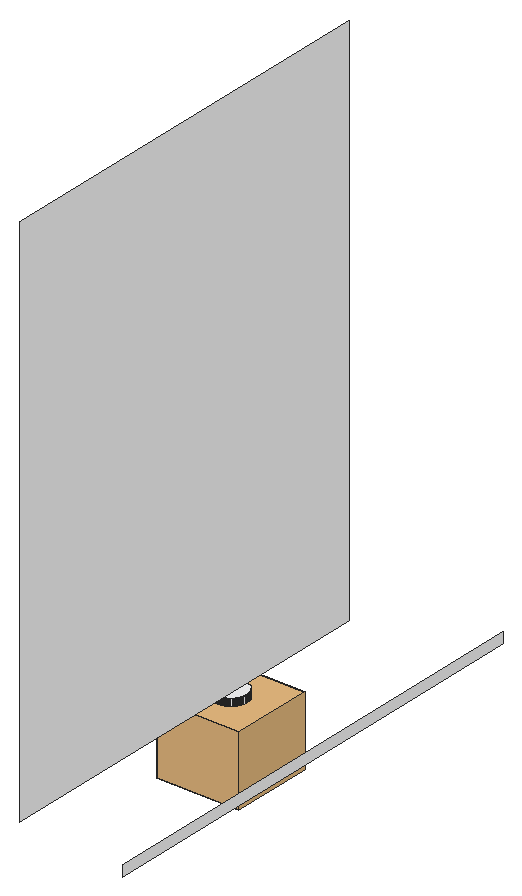
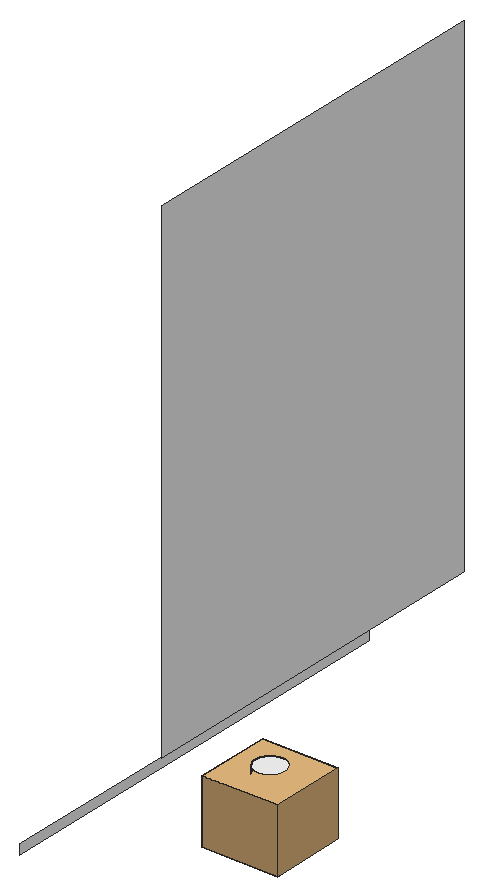
# SketchUp Ruby script. Lengths in inches.
U = 1.inch
M = Sketchup.active_model
def pt(a) = Geom::Point3d.new(a.map { |v| v * U })
def face(e, loops, mat)
  f = e.add_face(loops[0].map { |a| pt(a) })
  loops[1..].each { |l| e.add_face(l.map { |a| pt(a) }).erase! }
  f.material = f.back_material = mat if mat
  f
end
# faces: each face lists its corners as indices into pts; further lists are holes
def faces(e, pts, list, mat = nil) = list.each { |f| face(e, (f[0].is_a?(Array) ? f : [f]).map { |l| l.map { |i| pts[i] } }, mat) }
# xy, xz, yz: faces in a plane at the given z, y or x. An outline is a flat list of corners, or four numbers for a rectangle; further outlines are holes
def ring(l) = l.size == 4 ? [[l[0], l[1]], [l[2], l[1]], [l[2], l[3]], [l[0], l[3]]] : l.each_slice(2).to_a
def flat(e, list, mat, &to3) = list.each { |f| face(e, (f[0].is_a?(Array) ? f : [f]).map { |l| ring(l).map { |u, v| to3.(u, v) } }, mat) }
def xy(e, z, list, mat = nil) = flat(e, list, mat) { |x, y| [x, y, z] }
def xz(e, y, list, mat = nil) = flat(e, list, mat) { |x, z| [x, y, z] }
def yz(e, x, list, mat = nil) = flat(e, list, mat) { |y, z| [x, y, z] }
def lines(e, pts, list) = list.each { |a, b| e.add_line(pt(pts[a]), pt(pts[b])) }
# prism: a flat outline (further loops are holes) pulled along v
def prism(e, loops, v, mat = nil)
  f = face(e, loops, mat); d = Geom::Vector3d.new(v.map { |x| x * U })
  f.pushpull(f.normal.samedirection?(d) ? d.length : -d.length)
end
def box(e, o, s, mat = nil) = prism(e, [[o, [o[0] + s[0], o[1], o[2]], [o[0] + s[0], o[1] + s[1], o[2]], [o[0], o[1] + s[1], o[2]]]], [0, 0, s[2]], mat)
def at(x, y, z, deg = 0) = Geom::Transformation.translation(pt([x, y, z])) * Geom::Transformation.rotation(ORIGIN, Z_AXIS, deg.degrees)
def axes(o, x, y, z) = Geom::Transformation.new([*x, 0, *y, 0, *z, 0, *pt(o).to_a, 1])
def part(name) = M.definitions.add(name)
# library, detail: a bought-in or finely detailed component or shape, given as its bounding box
def library(name, o, s) = part(name).tap { |d| box(d.entities, o, s) }
def detail(e, o, s) = box(e.add_group.entities, o, s)
def put(e, d, t, mat = nil) = e.add_instance(d, t).tap { |i| i.material = mat if mat }
def group(e, t, mat = nil) = e.add_group.tap { |g| g.transformation = t; g.material = mat if mat }.entities
root = M.entities
M.materials.add("[Quartz Light Grey]").color = [251, 251, 252]
c1 = library("5",[-6.25,-6.25,-13.16],[15.58,15.58,13.16])
xy(root,119.5,[[207.84,250,207.76,250.01,207.6875,250.02,207.61,250.03,207.45,250.05,207.375,250.07,207.3,250.08,207.22,250.1,207.15,250.125,207.07,250.15,207,250.17,206.92,250.2,206.71,250.29,206.64,250.33,206.57,250.36,206.43,250.44,206.37,250.48,206.3,250.53,206.24,250.57,206.17,250.62,205.93,250.82,205.88,250.88,205.82,250.93,205.62,251.17,205.57,251.24,205.53,251.3,205.48,251.37,205.44,251.43,205.36,251.57,205.33,251.64,205.29,251.71,205.2,251.92,205.17,252,205.15,252.07,205.125,252.15,205.1,252.22,205.08,252.3,205.07,252.375,205.05,252.45,205.03,252.61,205.02,252.6875,205.01,252.76,205,252.84,205,253.16,205.01,253.24,205.02,253.3125,205.03,253.39,205.05,253.55,205.07,253.625,205.08,253.7,205.1,253.78,205.125,253.85,205.15,253.93,205.17,254,205.2,254.08,205.29,254.29,205.33,254.36,205.36,254.43,205.44,254.57,205.48,254.63,205.53,254.7,205.57,254.76,205.62,254.83,205.82,255.07,205.88,255.12,205.93,255.18,206.17,255.38,206.24,255.43,206.3,255.47,206.37,255.52,206.43,255.56,206.57,255.64,206.64,255.67,206.71,255.71,206.92,255.8,207,255.83,207.07,255.85,207.15,255.875,207.22,255.9,207.3,255.92,207.375,255.93,207.45,255.95,207.61,255.97,207.6875,255.98,207.76,255.99,207.84,256,208.16,256,208.24,255.99,208.3125,255.98,208.39,255.97,208.55,255.95,208.625,255.93,208.7,255.92,208.78,255.9,208.85,255.875,208.93,255.85,209,255.83,209.08,255.8,209.29,255.71,209.36,255.67,209.43,255.64,209.57,255.56,209.63,255.52,209.7,255.47,209.76,255.43,209.83,255.38,210.07,255.18,210.12,255.12,210.18,255.07,210.38,254.83,210.43,254.76,210.47,254.7,210.52,254.63,210.56,254.57,210.64,254.43,210.67,254.36,210.71,254.29,210.8,254.08,210.83,254,210.85,253.93,210.875,253.85,210.9,253.78,210.92,253.7,210.93,253.625,210.95,253.55,210.97,253.39,210.98,253.3125,210.99,253.24,211,253.16,211,252.84,210.99,252.76,210.98,252.6875,210.97,252.61,210.95,252.45,210.93,252.375,210.92,252.3,210.9,252.22,210.875,252.15,210.85,252.07,210.83,252,210.8,251.92,210.71,251.71,210.67,251.64,210.64,251.57,210.56,251.43,210.52,251.37,210.47,251.3,210.43,251.24,210.38,251.17,210.18,250.93,210.12,250.88,210.07,250.82,209.83,250.62,209.76,250.57,209.7,250.53,209.63,250.48,209.57,250.44,209.43,250.36,209.36,250.33,209.29,250.29,209.08,250.2,209,250.17,208.93,250.15,208.85,250.125,208.78,250.1,208.7,250.08,208.625,250.07,208.55,250.05,208.39,250.03,208.3125,250.02,208.24,250.01,208.16,250]],"[Quartz Light Grey]")
xz(root,250,[[207.84,117,207.92,119.5],[207.92,117,208,119.5],[208,117,208.08,119.5],[208.08,117,208.16,119.5]],"[Quartz Light Grey]")
yz(root,211,[[252.84,117,252.92,119.5],[252.92,117,253,119.5],[253,117,253.08,119.5],[253.08,117,253.16,119.5]],"[Quartz Light Grey]")
yz(root,216,[[193,126,271,228]],"[Quartz Light Grey]")
yz(root,226,[[205,115,295,117]],"[Quartz Light Grey]")
p = [[207.53,250.04,117],[207.45,250.05,117],[207.45,250.05,119.5],[207.53,250.04,119.5],[207.61,250.03,117],[207.61,250.03,119.5],
  [207.6875,250.02,117],[207.6875,250.02,119.5],[207.76,250.01,117],[207.76,250.01,119.5],[207.84,250,117],[207.84,250,119.5],
  [208.24,250.01,117],[208.16,250,117],[208.16,250,119.5],[208.24,250.01,119.5],[208.3125,250.02,117],[208.3125,250.02,119.5],
  [208.39,250.03,117],[208.39,250.03,119.5],[208.47,250.04,117],[208.47,250.04,119.5],[208.55,250.05,117],[208.55,250.05,119.5],
  [207.3,250.08,117],[207.22,250.1,117],[207.22,250.1,119.5],[207.3,250.08,119.5],[207.375,250.07,117],[207.375,250.07,119.5],
  [208.625,250.07,117],[208.625,250.07,119.5],[208.7,250.08,117],[208.7,250.08,119.5],[208.78,250.1,117],[208.78,250.1,119.5],
  [208.85,250.125,117],[208.85,250.125,119.5],[208.93,250.15,117],[208.93,250.15,119.5],[209,250.17,117],[209,250.17,119.5],
  [209.08,250.2,117],[209.08,250.2,119.5],[209.15,250.23,117],[209.15,250.23,119.5],[209.22,250.26,117],[209.22,250.26,119.5],
  [209.29,250.29,117],[209.29,250.29,119.5],[209.36,250.33,117],[209.36,250.33,119.5],[209.43,250.36,117],[209.43,250.36,119.5],
  [209.5,250.4,117],[209.5,250.4,119.5],[209.57,250.44,117],[209.57,250.44,119.5],[209.63,250.48,117],[209.63,250.48,119.5],
  [209.7,250.53,117],[209.7,250.53,119.5],[209.76,250.57,117],[209.76,250.57,119.5],[209.83,250.62,117],[209.83,250.62,119.5],
  [209.89,250.67,117],[209.89,250.67,119.5],[209.95,250.72,117],[209.95,250.72,119.5],[210.01,250.77,117],[210.01,250.77,119.5],
  [210.07,250.82,117],[210.07,250.82,119.5],[210.12,250.88,117],[210.12,250.88,119.5],[210.18,250.93,117],[210.18,250.93,119.5],
  [210.23,250.99,117],[210.23,250.99,119.5],[210.28,251.05,117],[210.28,251.05,119.5],[210.33,251.11,117],[210.33,251.11,119.5],
  [210.38,251.17,117],[210.38,251.17,119.5],[210.43,251.24,117],[210.43,251.24,119.5],[210.47,251.3,117],[210.47,251.3,119.5],
  [210.52,251.37,117],[210.52,251.37,119.5],[210.56,251.43,117],[210.56,251.43,119.5],[210.6,251.5,117],[210.6,251.5,119.5],
  [210.64,251.57,117],[210.64,251.57,119.5],[210.67,251.64,117],[210.67,251.64,119.5],[210.71,251.71,117],[210.71,251.71,119.5],
  [210.74,251.78,117],[210.74,251.78,119.5],[210.77,251.85,117],[210.77,251.85,119.5],[210.8,251.92,117],[210.8,251.92,119.5],
  [210.83,252,117],[210.83,252,119.5],[210.85,252.07,117],[210.85,252.07,119.5],[210.875,252.15,117],[210.875,252.15,119.5],
  [210.9,252.22,117],[210.9,252.22,119.5],[210.92,252.3,117],[210.92,252.3,119.5],[210.93,252.375,117],[210.93,252.375,119.5],
  [210.95,252.45,117],[210.95,252.45,119.5],[210.96,252.53,117],[210.96,252.53,119.5],[210.97,252.61,117],[210.97,252.61,119.5],
  [210.98,252.6875,117],[210.98,252.6875,119.5],[210.99,252.76,117],[210.99,252.76,119.5],[211,252.84,117],[211,252.84,119.5],
  [210.98,253.3125,117],[210.99,253.24,117],[210.99,253.24,119.5],[210.98,253.3125,119.5],[211,253.16,117],[211,253.16,119.5],
  [210.97,253.39,117],[210.97,253.39,119.5],[210.96,253.47,117],[210.96,253.47,119.5],[210.93,253.625,117],[210.95,253.55,117],
  [210.95,253.55,119.5],[210.93,253.625,119.5],[210.92,253.7,117],[210.92,253.7,119.5],[210.9,253.78,117],[210.9,253.78,119.5],
  [210.875,253.85,117],[210.875,253.85,119.5],[210.83,254,117],[210.85,253.93,117],[210.85,253.93,119.5],[210.83,254,119.5],
  [210.8,254.08,117],[210.8,254.08,119.5],[210.74,254.22,117],[210.77,254.15,117],[210.77,254.15,119.5],[210.74,254.22,119.5],
  [210.71,254.29,117],[210.71,254.29,119.5],[210.67,254.36,117],[210.67,254.36,119.5],[210.6,254.5,117],[210.64,254.43,117],
  [210.64,254.43,119.5],[210.6,254.5,119.5],[210.56,254.57,117],[210.56,254.57,119.5],[210.47,254.7,117],[210.52,254.63,117],
  [210.52,254.63,119.5],[210.47,254.7,119.5],[210.43,254.76,117],[210.43,254.76,119.5],[210.33,254.89,117],[210.38,254.83,117],
  [210.38,254.83,119.5],[210.33,254.89,119.5]]
faces(root,p,[[0,1,2,3],[4,0,3,5],[6,4,5,7],[8,6,7,9],[10,8,9,11],[12,13,14,15],[16,12,15,17],[18,16,17,19],
  [20,18,19,21],[22,20,21,23],[24,25,26,27],[28,24,27,29],[1,28,29,2],[30,22,23,31],[32,30,31,33],[34,32,33,35],
  [36,34,35,37],[38,36,37,39],[40,38,39,41],[42,40,41,43],[44,42,43,45],[46,44,45,47],[48,46,47,49],[50,48,49,51],
  [52,50,51,53],[54,52,53,55],[56,54,55,57],[58,56,57,59],[60,58,59,61],[62,60,61,63],[64,62,63,65],[66,64,65,67],
  [68,66,67,69],[70,68,69,71],[72,70,71,73],[74,72,73,75],[76,74,75,77],[78,76,77,79],[80,78,79,81],[82,80,81,83],
  [84,82,83,85],[86,84,85,87],[88,86,87,89],[90,88,89,91],[92,90,91,93],[94,92,93,95],[96,94,95,97],[98,96,97,99],
  [100,98,99,101],[102,100,101,103],[104,102,103,105],[106,104,105,107],[108,106,107,109],[110,108,109,111],[112,110,111,113],[114,112,113,115],
  [116,114,115,117],[118,116,117,119],[120,118,119,121],[122,120,121,123],[124,122,123,125],[126,124,125,127],[128,126,127,129],[130,128,129,131],
  [132,133,134,135],[133,136,137,134],[138,132,135,139],[140,138,139,141],[142,143,144,145],[143,140,141,144],[146,142,145,147],[148,146,147,149],
  [150,148,149,151],[152,153,154,155],[153,150,151,154],[156,152,155,157],[158,159,160,161],[159,156,157,160],[162,158,161,163],[164,162,163,165],
  [166,167,168,169],[167,164,165,168],[170,166,169,171],[172,173,174,175],[173,170,171,174],[176,172,175,177],[178,179,180,181],[179,176,177,180]],"[Quartz Light Grey]")
put(root,c1,at(206.46,251.46,118.25),"[Quartz Light Grey]")
